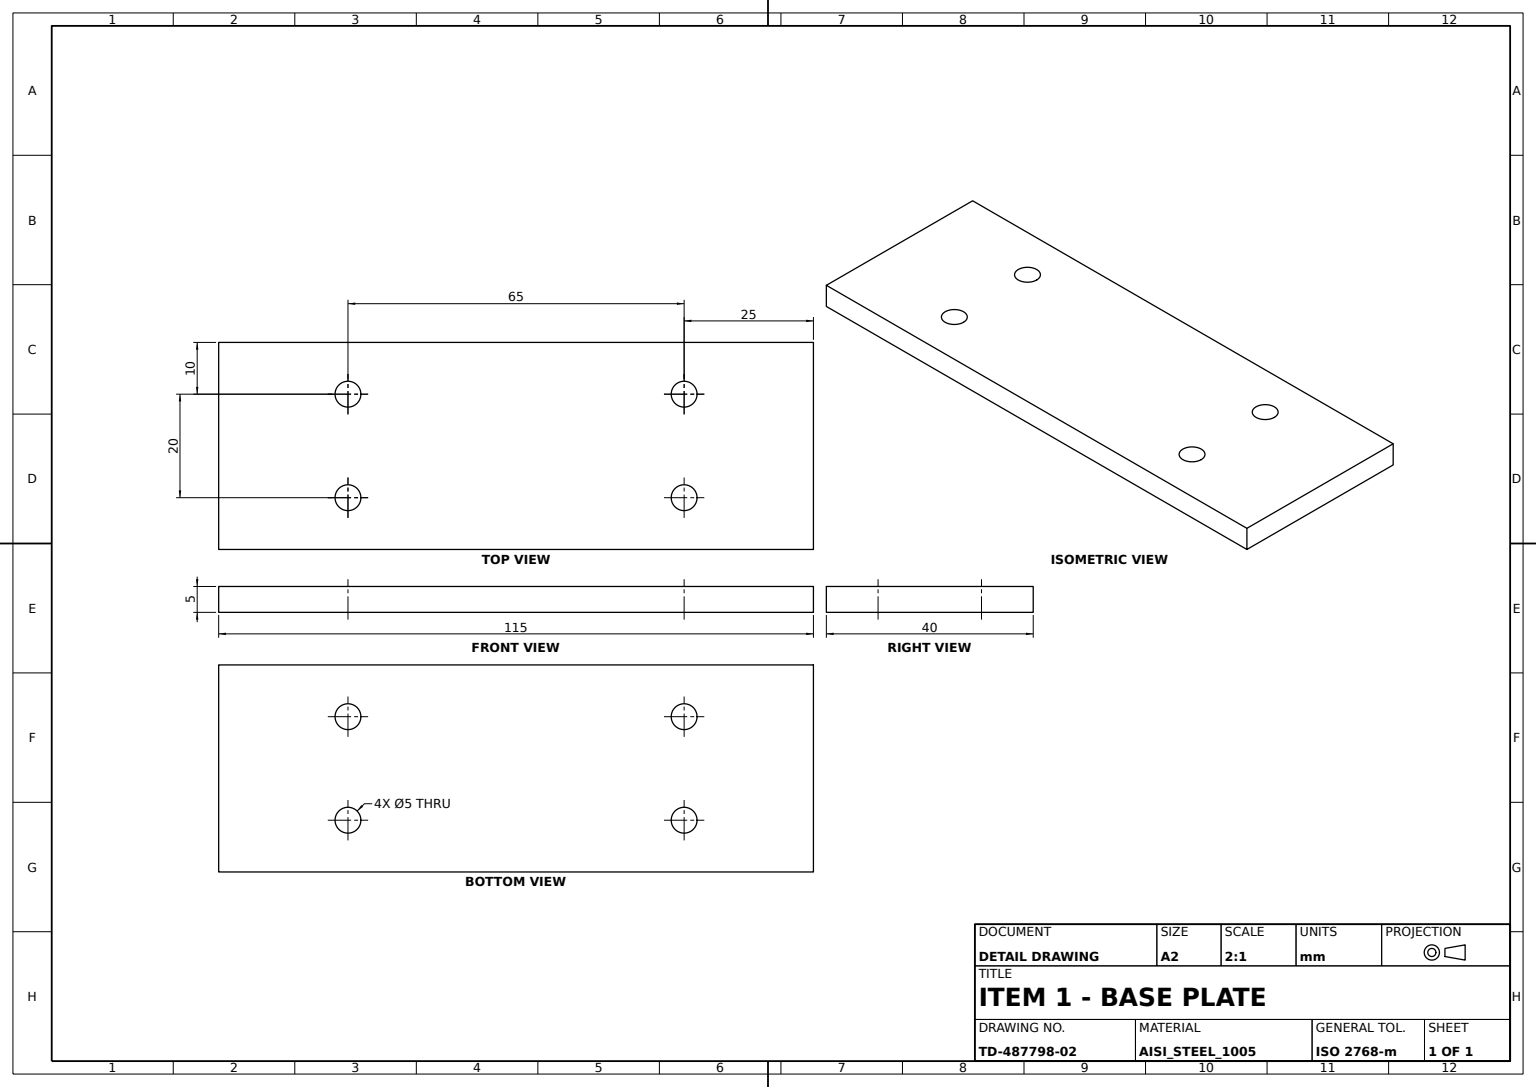
ISO-10303-21;
HEADER;
FILE_DESCRIPTION((''),'2;1');
FILE_NAME('','',(''),(''),'','','');
FILE_SCHEMA(('AUTOMOTIVE_DESIGN'));
ENDSEC;
DATA;
#1=APPLICATION_CONTEXT('');
#2=PRODUCT_CONTEXT('',#1,'mechanical');
#3=PRODUCT('','','',(#2));
#4=PRODUCT_DEFINITION_FORMATION('','',#3);
#5=PRODUCT_DEFINITION_CONTEXT('',#1,'design');
#6=PRODUCT_DEFINITION('','',#4,#5);
#7=PRODUCT_DEFINITION_SHAPE('','',#6);
#8=(LENGTH_UNIT()NAMED_UNIT(*)SI_UNIT(.MILLI.,.METRE.));
#9=(NAMED_UNIT(*)PLANE_ANGLE_UNIT()SI_UNIT($,.RADIAN.));
#10=(NAMED_UNIT(*)SI_UNIT($,.STERADIAN.)SOLID_ANGLE_UNIT());
#11=UNCERTAINTY_MEASURE_WITH_UNIT(LENGTH_MEASURE(0.005),#8,'distance_accuracy_value','');
#12=(GEOMETRIC_REPRESENTATION_CONTEXT(3)GLOBAL_UNCERTAINTY_ASSIGNED_CONTEXT((#11))GLOBAL_UNIT_ASSIGNED_CONTEXT((#8,#9,#10))REPRESENTATION_CONTEXT('',''));
#13=CARTESIAN_POINT('',(-30.,-10.,0.));
#14=VERTEX_POINT('',#13);
#15=CARTESIAN_POINT('',(-32.5,-10.,0.));
#16=DIRECTION('',(0.,0.,1.));
#17=DIRECTION('',(1.,0.,0.));
#18=AXIS2_PLACEMENT_3D('',#15,#16,#17);
#19=CIRCLE('',#18,2.5);
#20=EDGE_CURVE('',#14,#14,#19,.T.);
#21=ORIENTED_EDGE('',*,*,#20,.F.);
#22=EDGE_LOOP('',(#21));
#23=FACE_BOUND('',#22,.T.);
#24=CARTESIAN_POINT('',(-30.,-10.,5.));
#25=VERTEX_POINT('',#24);
#26=CARTESIAN_POINT('',(-32.5,-10.,5.));
#27=AXIS2_PLACEMENT_3D('',#26,#16,#17);
#28=CIRCLE('',#27,2.5);
#29=EDGE_CURVE('',#25,#25,#28,.T.);
#30=ORIENTED_EDGE('',*,*,#29,.T.);
#31=EDGE_LOOP('',(#30));
#32=FACE_BOUND('',#31,.T.);
#33=DIRECTION('',(0.,0.,-1.));
#34=DIRECTION('',(-1.,0.,0.));
#35=AXIS2_PLACEMENT_3D('',#26,#33,#34);
#36=CYLINDRICAL_SURFACE('',#35,2.5);
#37=ADVANCED_FACE('',(#23,#32),#36,.F.);
#38=CARTESIAN_POINT('',(35.,-10.,5.));
#39=VERTEX_POINT('',#38);
#40=CARTESIAN_POINT('',(32.5,-10.,5.));
#41=AXIS2_PLACEMENT_3D('',#40,#16,#17);
#42=CIRCLE('',#41,2.5);
#43=EDGE_CURVE('',#39,#39,#42,.T.);
#44=ORIENTED_EDGE('',*,*,#43,.T.);
#45=EDGE_LOOP('',(#44));
#46=FACE_BOUND('',#45,.T.);
#47=CARTESIAN_POINT('',(35.,-10.,0.));
#48=VERTEX_POINT('',#47);
#49=CARTESIAN_POINT('',(32.5,-10.,0.));
#50=AXIS2_PLACEMENT_3D('',#49,#16,#17);
#51=CIRCLE('',#50,2.5);
#52=EDGE_CURVE('',#48,#48,#51,.T.);
#53=ORIENTED_EDGE('',*,*,#52,.F.);
#54=EDGE_LOOP('',(#53));
#55=FACE_BOUND('',#54,.T.);
#56=AXIS2_PLACEMENT_3D('',#40,#33,#34);
#57=CYLINDRICAL_SURFACE('',#56,2.5);
#58=ADVANCED_FACE('',(#46,#55),#57,.F.);
#59=CARTESIAN_POINT('',(35.,10.,5.));
#60=VERTEX_POINT('',#59);
#61=CARTESIAN_POINT('',(32.5,10.,5.));
#62=AXIS2_PLACEMENT_3D('',#61,#16,#17);
#63=CIRCLE('',#62,2.5);
#64=EDGE_CURVE('',#60,#60,#63,.T.);
#65=ORIENTED_EDGE('',*,*,#64,.T.);
#66=EDGE_LOOP('',(#65));
#67=FACE_BOUND('',#66,.T.);
#68=CARTESIAN_POINT('',(35.,10.,0.));
#69=VERTEX_POINT('',#68);
#70=CARTESIAN_POINT('',(32.5,10.,0.));
#71=AXIS2_PLACEMENT_3D('',#70,#16,#17);
#72=CIRCLE('',#71,2.5);
#73=EDGE_CURVE('',#69,#69,#72,.T.);
#74=ORIENTED_EDGE('',*,*,#73,.F.);
#75=EDGE_LOOP('',(#74));
#76=FACE_BOUND('',#75,.T.);
#77=AXIS2_PLACEMENT_3D('',#61,#33,#34);
#78=CYLINDRICAL_SURFACE('',#77,2.5);
#79=ADVANCED_FACE('',(#67,#76),#78,.F.);
#80=CARTESIAN_POINT('',(57.5,-20.,5.));
#81=VERTEX_POINT('',#80);
#82=CARTESIAN_POINT('',(57.5,-20.,0.));
#83=VERTEX_POINT('',#82);
#84=VECTOR('',#33,1000.);
#85=LINE('',#80,#84);
#86=EDGE_CURVE('',#81,#83,#85,.T.);
#87=ORIENTED_EDGE('',*,*,#86,.F.);
#88=CARTESIAN_POINT('',(-57.5,-20.,5.));
#89=VERTEX_POINT('',#88);
#90=VECTOR('',#34,1000.);
#91=LINE('',#80,#90);
#92=EDGE_CURVE('',#81,#89,#91,.T.);
#93=ORIENTED_EDGE('',*,*,#92,.T.);
#94=CARTESIAN_POINT('',(-57.5,-20.,0.));
#95=VERTEX_POINT('',#94);
#96=LINE('',#88,#84);
#97=EDGE_CURVE('',#89,#95,#96,.T.);
#98=ORIENTED_EDGE('',*,*,#97,.T.);
#99=LINE('',#82,#90);
#100=EDGE_CURVE('',#83,#95,#99,.T.);
#101=ORIENTED_EDGE('',*,*,#100,.F.);
#102=EDGE_LOOP('',(#87,#93,#98,#101));
#103=FACE_BOUND('',#102,.T.);
#104=DIRECTION('',(0.,-1.,0.));
#105=AXIS2_PLACEMENT_3D('',#80,#104,#33);
#106=PLANE('',#105);
#107=ADVANCED_FACE('',(#103),#106,.T.);
#108=CARTESIAN_POINT('',(57.5,20.,0.));
#109=VERTEX_POINT('',#108);
#110=VECTOR('',#104,1000.);
#111=LINE('',#108,#110);
#112=EDGE_CURVE('',#109,#83,#111,.T.);
#113=ORIENTED_EDGE('',*,*,#112,.F.);
#114=CARTESIAN_POINT('',(57.5,20.,5.));
#115=VERTEX_POINT('',#114);
#116=LINE('',#114,#84);
#117=EDGE_CURVE('',#115,#109,#116,.T.);
#118=ORIENTED_EDGE('',*,*,#117,.F.);
#119=LINE('',#114,#110);
#120=EDGE_CURVE('',#115,#81,#119,.T.);
#121=ORIENTED_EDGE('',*,*,#120,.T.);
#122=ORIENTED_EDGE('',*,*,#86,.T.);
#123=EDGE_LOOP('',(#113,#118,#121,#122));
#124=FACE_BOUND('',#123,.T.);
#125=DIRECTION('',(0.,1.,0.));
#126=AXIS2_PLACEMENT_3D('',#114,#17,#125);
#127=PLANE('',#126);
#128=ADVANCED_FACE('',(#124),#127,.T.);
#129=ORIENTED_EDGE('',*,*,#120,.F.);
#130=CARTESIAN_POINT('',(-57.5,20.,5.));
#131=VERTEX_POINT('',#130);
#132=VECTOR('',#17,1000.);
#133=LINE('',#130,#132);
#134=EDGE_CURVE('',#131,#115,#133,.T.);
#135=ORIENTED_EDGE('',*,*,#134,.F.);
#136=VECTOR('',#125,1000.);
#137=LINE('',#88,#136);
#138=EDGE_CURVE('',#89,#131,#137,.T.);
#139=ORIENTED_EDGE('',*,*,#138,.F.);
#140=ORIENTED_EDGE('',*,*,#92,.F.);
#141=EDGE_LOOP('',(#129,#135,#139,#140));
#142=FACE_BOUND('',#141,.T.);
#143=ORIENTED_EDGE('',*,*,#64,.F.);
#144=EDGE_LOOP('',(#143));
#145=FACE_BOUND('',#144,.T.);
#146=ORIENTED_EDGE('',*,*,#29,.F.);
#147=EDGE_LOOP('',(#146));
#148=FACE_BOUND('',#147,.T.);
#149=CARTESIAN_POINT('',(-30.,10.,5.));
#150=VERTEX_POINT('',#149);
#151=CARTESIAN_POINT('',(-32.5,10.,5.));
#152=AXIS2_PLACEMENT_3D('',#151,#16,#17);
#153=CIRCLE('',#152,2.5);
#154=EDGE_CURVE('',#150,#150,#153,.T.);
#155=ORIENTED_EDGE('',*,*,#154,.F.);
#156=EDGE_LOOP('',(#155));
#157=FACE_BOUND('',#156,.T.);
#158=ORIENTED_EDGE('',*,*,#43,.F.);
#159=EDGE_LOOP('',(#158));
#160=FACE_BOUND('',#159,.T.);
#161=PLANE('',#62);
#162=ADVANCED_FACE('',(#142,#145,#148,#157,#160),#161,.T.);
#163=ORIENTED_EDGE('',*,*,#52,.T.);
#164=EDGE_LOOP('',(#163));
#165=FACE_BOUND('',#164,.T.);
#166=CARTESIAN_POINT('',(-30.,10.,0.));
#167=VERTEX_POINT('',#166);
#168=CARTESIAN_POINT('',(-32.5,10.,0.));
#169=AXIS2_PLACEMENT_3D('',#168,#16,#17);
#170=CIRCLE('',#169,2.5);
#171=EDGE_CURVE('',#167,#167,#170,.T.);
#172=ORIENTED_EDGE('',*,*,#171,.T.);
#173=EDGE_LOOP('',(#172));
#174=FACE_BOUND('',#173,.T.);
#175=ORIENTED_EDGE('',*,*,#20,.T.);
#176=EDGE_LOOP('',(#175));
#177=FACE_BOUND('',#176,.T.);
#178=ORIENTED_EDGE('',*,*,#73,.T.);
#179=EDGE_LOOP('',(#178));
#180=FACE_BOUND('',#179,.T.);
#181=CARTESIAN_POINT('',(-57.5,20.,0.));
#182=VERTEX_POINT('',#181);
#183=LINE('',#94,#136);
#184=EDGE_CURVE('',#95,#182,#183,.T.);
#185=ORIENTED_EDGE('',*,*,#184,.T.);
#186=LINE('',#181,#132);
#187=EDGE_CURVE('',#182,#109,#186,.T.);
#188=ORIENTED_EDGE('',*,*,#187,.T.);
#189=ORIENTED_EDGE('',*,*,#112,.T.);
#190=ORIENTED_EDGE('',*,*,#100,.T.);
#191=EDGE_LOOP('',(#185,#188,#189,#190));
#192=FACE_BOUND('',#191,.T.);
#193=PLANE('',#71);
#194=ADVANCED_FACE('',(#165,#174,#177,#180,#192),#193,.F.);
#195=LINE('',#130,#84);
#196=EDGE_CURVE('',#131,#182,#195,.T.);
#197=ORIENTED_EDGE('',*,*,#196,.F.);
#198=ORIENTED_EDGE('',*,*,#134,.T.);
#199=ORIENTED_EDGE('',*,*,#117,.T.);
#200=ORIENTED_EDGE('',*,*,#187,.F.);
#201=EDGE_LOOP('',(#197,#198,#199,#200));
#202=FACE_BOUND('',#201,.T.);
#203=AXIS2_PLACEMENT_3D('',#130,#125,#16);
#204=PLANE('',#203);
#205=ADVANCED_FACE('',(#202),#204,.T.);
#206=ORIENTED_EDGE('',*,*,#154,.T.);
#207=EDGE_LOOP('',(#206));
#208=FACE_BOUND('',#207,.T.);
#209=ORIENTED_EDGE('',*,*,#171,.F.);
#210=EDGE_LOOP('',(#209));
#211=FACE_BOUND('',#210,.T.);
#212=AXIS2_PLACEMENT_3D('',#151,#33,#34);
#213=CYLINDRICAL_SURFACE('',#212,2.5);
#214=ADVANCED_FACE('',(#208,#211),#213,.F.);
#215=ORIENTED_EDGE('',*,*,#184,.F.);
#216=ORIENTED_EDGE('',*,*,#97,.F.);
#217=ORIENTED_EDGE('',*,*,#138,.T.);
#218=ORIENTED_EDGE('',*,*,#196,.T.);
#219=EDGE_LOOP('',(#215,#216,#217,#218));
#220=FACE_BOUND('',#219,.T.);
#221=AXIS2_PLACEMENT_3D('',#88,#34,#104);
#222=PLANE('',#221);
#223=ADVANCED_FACE('',(#220),#222,.T.);
#224=CLOSED_SHELL('',(#37,#58,#79,#107,#128,#162,#194,#205,#214,#223));
#225=MANIFOLD_SOLID_BREP('',#224);
#226=ADVANCED_BREP_SHAPE_REPRESENTATION('',(#225),#12);
#227=SHAPE_DEFINITION_REPRESENTATION(#7,#226);
ENDSEC;
END-ISO-10303-21;
